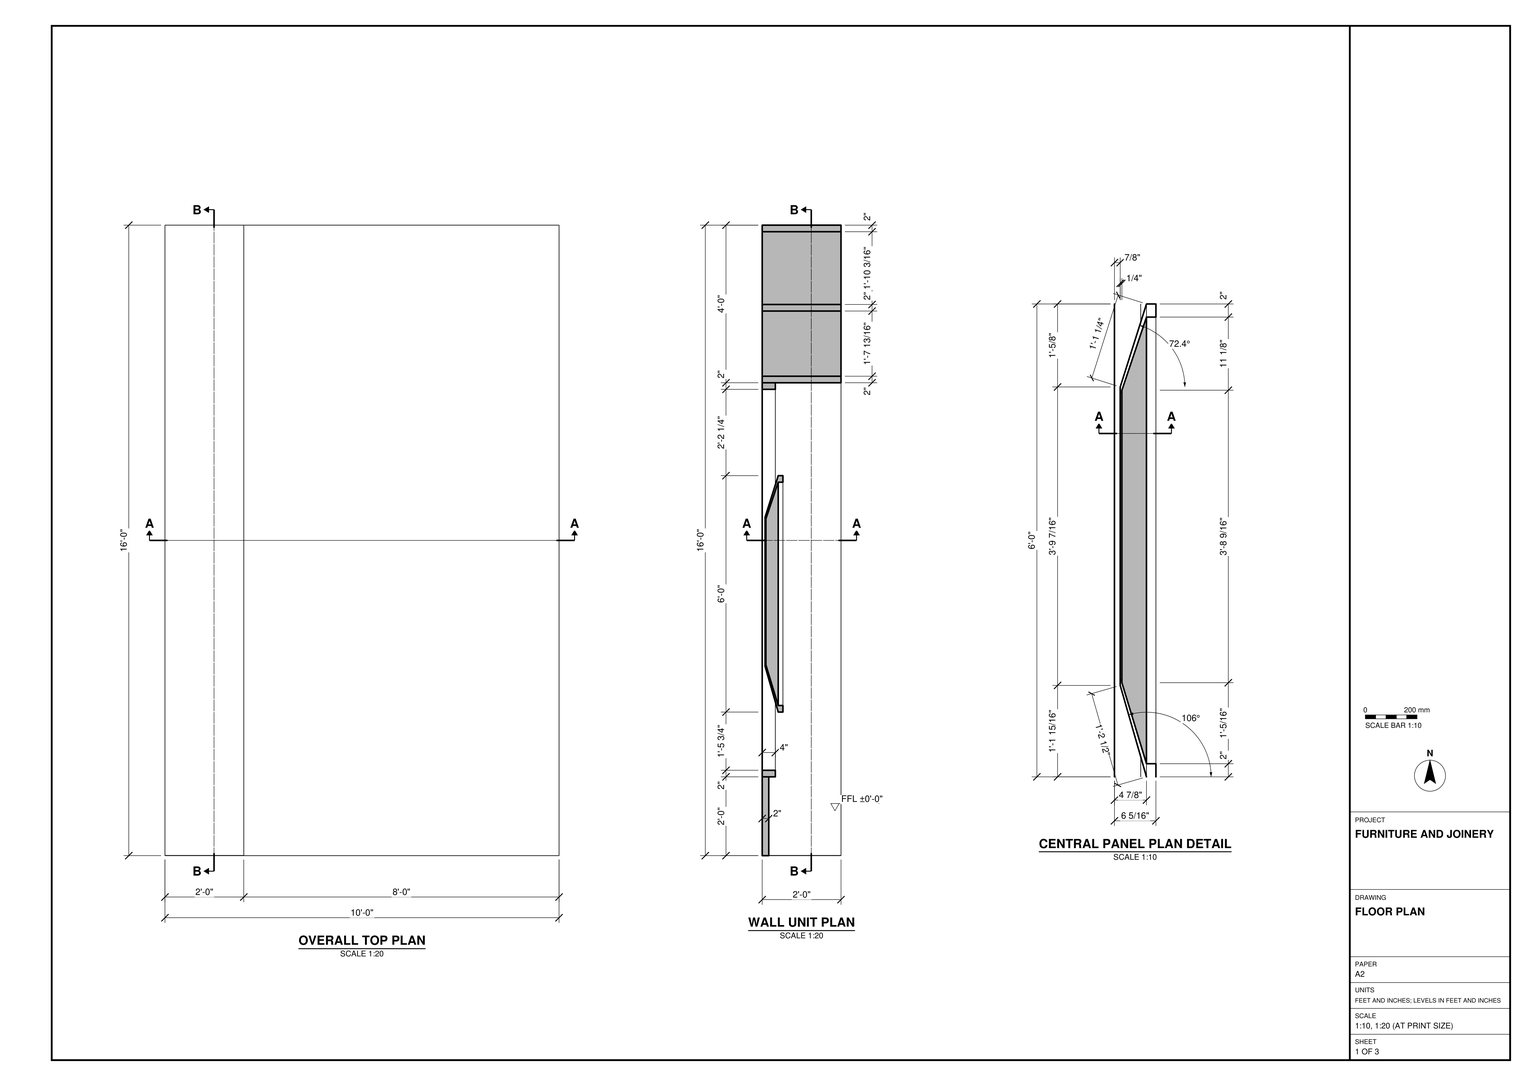
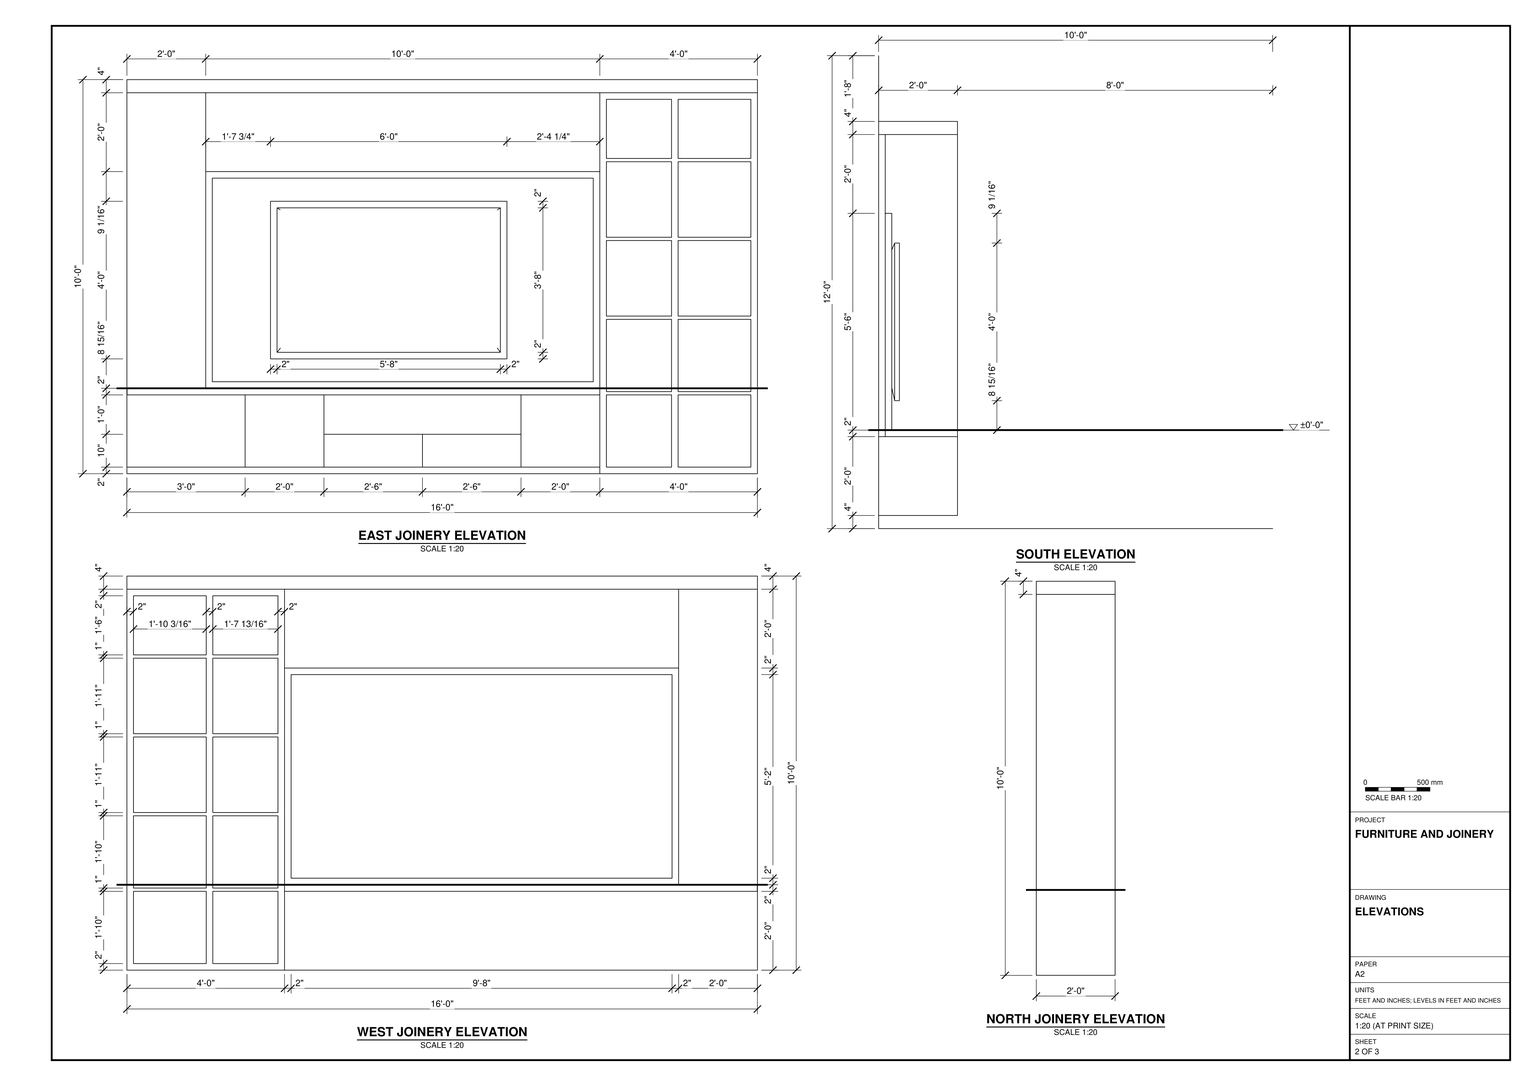
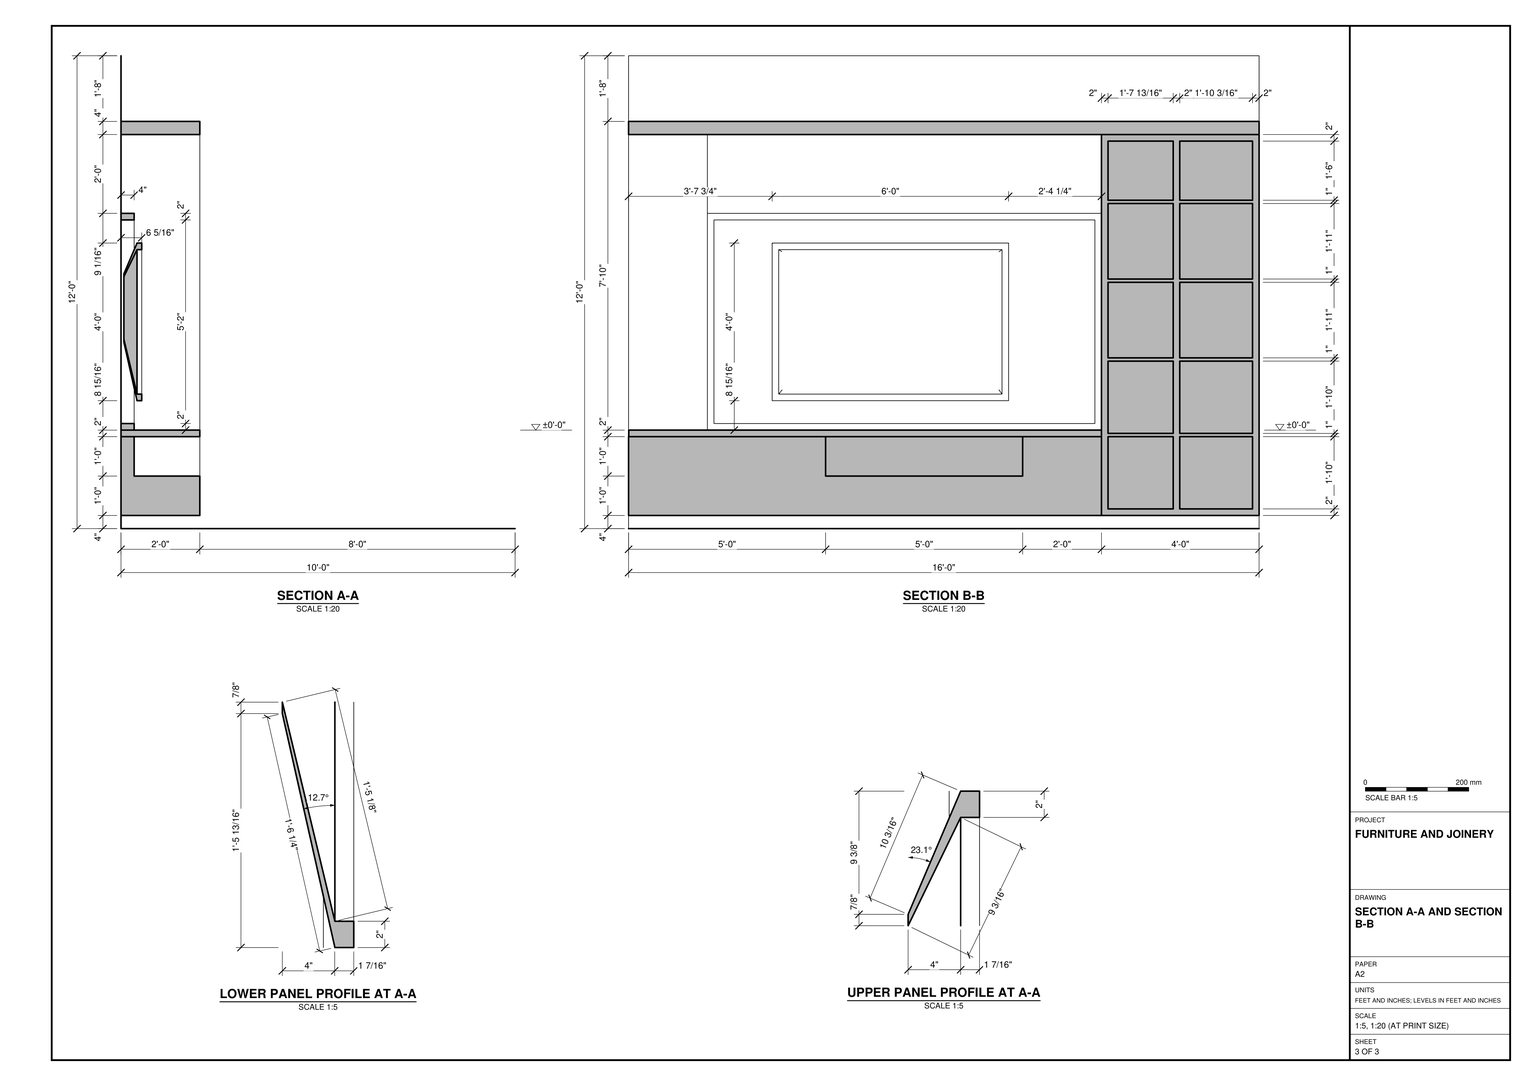
Model the wall unit and its surrounding extent in SketchUp using task_files/diagram_01.pdf. Work in feet and inches. The overall model is 10'-0" across X, 16'-0" along Y and 12'-0" high. Use the single finished-floor datum of ±0'-0" shown in the sections. The joinery itself is 10'-0" high and occupies a 2'-0" deep strip along one long edge of the plan.

Use the east elevation to lay out the plain end bay, framed central field and full-height shelving, in that order from left to right. Follow the elevation for the divisions in the low storage front, including the wide compartment above the divided lower pair. Model the smaller panel within the central field in three dimensions: use the plan detail for its angled ends and section A-A for its different upper and lower slopes. Use the west elevation to finish the reverse face rather than copying the east face. Match the thicknesses of the cap, shelves, dividers and frames to the drawings.

Keep the surrounding shell elements and the joinery in separate groups or components, and use components for repeated parts. Any decor or loose items shown may be represented by suitable library components. Save one SketchUp model as output_files/wall_unit_with_a_profiled_panel_and_shelving.skp.

# SketchUp Ruby script. Lengths in inches.
U = 1.inch
M = Sketchup.active_model
def pt(a) = Geom::Point3d.new(a.map { |v| v * U })
def face(e, loops, mat)
  f = e.add_face(loops[0].map { |a| pt(a) })
  loops[1..].each { |l| e.add_face(l.map { |a| pt(a) }).erase! }
  f.material = f.back_material = mat if mat
  f
end
# faces: each face lists its corners as indices into pts; further lists are holes
def faces(e, pts, list, mat = nil) = list.each { |f| face(e, (f[0].is_a?(Array) ? f : [f]).map { |l| l.map { |i| pts[i] } }, mat) }
# xy, xz, yz: faces in a plane at the given z, y or x. An outline is a flat list of corners, or four numbers for a rectangle; further outlines are holes
def ring(l) = l.size == 4 ? [[l[0], l[1]], [l[2], l[1]], [l[2], l[3]], [l[0], l[3]]] : l.each_slice(2).to_a
def flat(e, list, mat, &to3) = list.each { |f| face(e, (f[0].is_a?(Array) ? f : [f]).map { |l| ring(l).map { |u, v| to3.(u, v) } }, mat) }
def xy(e, z, list, mat = nil) = flat(e, list, mat) { |x, y| [x, y, z] }
def xz(e, y, list, mat = nil) = flat(e, list, mat) { |x, z| [x, y, z] }
def yz(e, x, list, mat = nil) = flat(e, list, mat) { |y, z| [x, y, z] }
def lines(e, pts, list) = list.each { |a, b| e.add_line(pt(pts[a]), pt(pts[b])) }
# prism: a flat outline (further loops are holes) pulled along v
def prism(e, loops, v, mat = nil)
  f = face(e, loops, mat); d = Geom::Vector3d.new(v.map { |x| x * U })
  f.pushpull(f.normal.samedirection?(d) ? d.length : -d.length)
end
def box(e, o, s, mat = nil) = prism(e, [[o, [o[0] + s[0], o[1], o[2]], [o[0] + s[0], o[1] + s[1], o[2]], [o[0], o[1] + s[1], o[2]]]], [0, 0, s[2]], mat)
def at(x, y, z, deg = 0) = Geom::Transformation.translation(pt([x, y, z])) * Geom::Transformation.rotation(ORIGIN, Z_AXIS, deg.degrees)
def axes(o, x, y, z) = Geom::Transformation.new([*x, 0, *y, 0, *z, 0, *pt(o).to_a, 1])
def part(name) = M.definitions.add(name)
# library, detail: a bought-in or finely detailed component or shape, given as its bounding box
def library(name, o, s) = part(name).tap { |d| box(d.entities, o, s) }
def detail(e, o, s) = box(e.add_group.entities, o, s)
def put(e, d, t, mat = nil) = e.add_instance(d, t).tap { |i| i.material = mat if mat }
def group(e, t, mat = nil) = e.add_group.tap { |g| g.transformation = t; g.material = mat if mat }.entities
root = M.entities
M.materials.add("[Color C01]").color = [255, 229, 204]
M.materials.add("[Color C08]").color = [102, 51, 0]
M.materials.add("[Color M09]").color = [0, 0, 0]
M.materials.add("[Tile Hexagon White]").color = [213, 206, 204]
M.materials.add("[Translucent Glass Gray]").color = [128, 128, 128]
M.materials["[Translucent Glass Gray]"].alpha = 0.5
M.materials.add("[Wood Cherry Original]").color = [152, 86, 42]
xy(root,0,[[0,0,120,192]])
xy(root,4,[[0,0,24,144],[0,144,24,192]])
xy(root,6,[[0,146,24,165.84],[0,167.84,24,190]],"[Color C01]")
xy(root,16,[[4,60,24,120]])
xy(root,28,[[0,0,2,0.0625],[2,0,24,0.0625],[0,0.0625,0,144,24,144,24,120,4,120,4,60,24,60,24,0.0625],[4,60,24,120]])
xy(root,28,[[0,146,24,165.84],[0,167.84,24,190]],"[Color C01]")
xy(root,29,[[0,146,24,165.84],[0,167.84,24,190]],"[Color C01]")
xy(root,30,[[0,0.0625,2,24],[0,24,4,144]])
xy(root,30,[[2,0.0625,24,0.0625,24,144,4,144,4,24,2,24]],"[Wood Cherry Original]")
xy(root,32,[[0,26,4,142]],"[Wood Cherry Original]")
xy(root,51,[[0,146,24,165.84],[0,167.84,24,190]],"[Color C01]")
xy(root,52,[[0,146,24,165.84],[0,167.84,24,190]],"[Color C01]")
xy(root,75,[[0,146,24,165.84],[0,167.84,24,190]],"[Color C01]")
xy(root,76,[[0,146,24,165.84],[0,167.84,24,190]],"[Color C01]")
xy(root,94,[[0,26,4,142]],"[Wood Cherry Original]")
xy(root,96,[[0,24,4,144]],"[Wood Cherry Original]")
xy(root,99,[[0,146,24,165.84],[0,167.84,24,190]],"[Color C01]")
xy(root,100,[[0,146,24,165.84],[0,167.84,24,190]],"[Color C01]")
xy(root,118,[[0,146,24,165.84],[0,167.84,24,190]],"[Color C01]")
xy(root,120,[[0,0,2,24],[0,144,24,192]])
xy(root,120,[[2,0,2,24,0,24,0,144,24,144,24,0]],"[Wood Cherry Original]")
xy(root,124,[[0,0,24,192]],"[Wood Cherry Original]")
xz(root,0,[[0,4,24,28]])
xz(root,0,[[0,28,2,120],[0,120,24,124]],"[Wood Cherry Original]")
xz(root,0.0625,[[0,28,2,30]])
xz(root,0.0625,[[2,28,24,30]],"[Wood Cherry Original]")
xz(root,24,[[0,30,2,96]])
xz(root,24,[[2,30,4,96],[0,96,2,120]],"[Wood Cherry Original]")
xz(root,26,[[0,32,4,94]],"[Wood Cherry Original]")
xz(root,60,[[4,16,24,28]])
xz(root,120,[[4,16,24,28]])
xz(root,142,[[0,32,4,94]],"[Wood Cherry Original]")
xz(root,144,[[0,4,24,28],[0,28,24,30],[0,30,4,96]])
xz(root,144,[[4,30,24,30,24,120,0,120,0,96,4,96]],"[Wood Cherry Original]")
xz(root,146,[[0,6,24,28],[0,29,24,51],[0,52,24,75],[0,76,24,99],[0,100,24,118]],"[Color C01]")
xz(root,165.84,[[0,6,24,28],[0,29,24,51],[0,52,24,75],[0,76,24,99],[0,100,24,118]],"[Color C01]")
xz(root,167.84,[[0,6,24,28],[0,29,24,51],[0,52,24,75],[0,76,24,99],[0,100,24,118]],"[Color C01]")
xz(root,190,[[0,6,24,28],[0,29,24,51],[0,52,24,75],[0,76,24,99],[0,100,24,118]],"[Color C01]")
xz(root,192,[[0,4,24,120]],"[Color C08]")
xz(root,192,[[0,120,24,124]],"[Wood Cherry Original]")
yz(root,0,[[0,0,192,4],[0,4,144,28],[[144,4,192,120],[167.84,52,190,75],[167.84,76,190,99],[167.84,29,190,51],[167.84,6,190,28],[146,76,165.84,99],[146,52,165.84,75],[146,6,165.84,28],[146,29,165.84,51],[167.84,100,190,118],[146,100,165.84,118]],[0,28,0,120,24,120,24,30,0.0625,30,0.0625,28],[0.0625,28,144,30],
  [[24,30,144,96],[26,32,142,94]],[0,120,192,124]])
yz(root,0,[[146,6,165.84,28],[167.84,6,190,28],[146,29,165.84,51],[167.84,29,190,51],[146,52,165.84,75],
  [167.84,52,190,75],[146,76,165.84,99],[167.84,76,190,99],[24,96,144,120],[146,100,165.84,118],
  [167.84,100,190,118],[0,124,192,144]],"[Color C01]")
yz(root,0,[[26,32,142,94]],"[Tile Hexagon White]")
yz(root,2,[[0,28,0.0625,28,0.0625,30,24,30,24,120,0,120]],"[Wood Cherry Original]")
yz(root,4,[[60,16,120,28]])
yz(root,4,[[[24,30,144,96],[26,32,142,94]]],"[Wood Cherry Original]")
yz(root,24,[[0,6,36,28],[36,6,60,28],[60,6,90,16],[90,6,120,16],[120,6,144,28]],"[Color C01]")
yz(root,24,[[[144,4,192,120],[167.84,52,190,75],[167.84,76,190,99],[167.84,29,190,51],[167.84,6,190,28],[146,76,165.84,99],[146,52,165.84,75],[146,29,165.84,51],[146,6,165.84,28],[167.84,100,190,118],[146,100,165.84,118]]],"[Color C08]")
yz(root,24,[[146,6,165.84,28],[167.84,6,190,28],[146,29,165.84,51],[167.84,29,190,51],[146,52,165.84,75],
  [167.84,52,190,75],[146,76,165.84,99],[167.84,76,190,99],[146,100,165.84,118],[167.84,100,190,118]],"[Translucent Glass Gray]")
yz(root,24,[[0,4,144,6],[0.0625,28,144,30],[0,120,192,124]],"[Wood Cherry Original]")
g1 = group(root,at(0.875,43.72,38.96),"[Color M09]")
xy(g1,0,[[4,0,5.4375,72]])
xy(g1,2,[[4,2,5.4375,70]])
xy(g1,46,[[4,2,5.4375,70]])
xy(g1,48,[[4,0,5.4375,72]])
xz(g1,0,[[4,0,5.4375,48]])
xz(g1,2,[[4,2,5.4375,46]])
xz(g1,70,[[4,2,5.4375,46]])
xz(g1,72,[[4,0,5.4375,48]])
yz(g1,0,[[[13.92,17.8125,59.36,38.62],[15.18,18.68,58.1,37.76]],[15.18,18.68,58.1,37.76]])
yz(g1,4,[[2,2,70,46]])
yz(g1,5.4375,[[[0,0,72,48],[2,2,70,46]]])
p = [[4,0,0],[0,13.92,17.8125],[0,59.36,17.8125],[4,72,0],[4,0,48],[0,13.92,38.62],
  [0,59.36,38.62],[4,72,48],[4,2,2],[0,15.18,18.68],[0,15.18,37.76],[4,2,46],
  [4,70,2],[0,58.1,18.68],[4,70,46],[0,58.1,37.76],[0,58.1,35.57]]
faces(g1,p,[[0,1,2,3],[4,5,1,0],[6,7,3,2],[8,9,10,11],[8,12,13,9],[13,12,14,15,16],[11,10,15,14],[4,7,6,5]])
